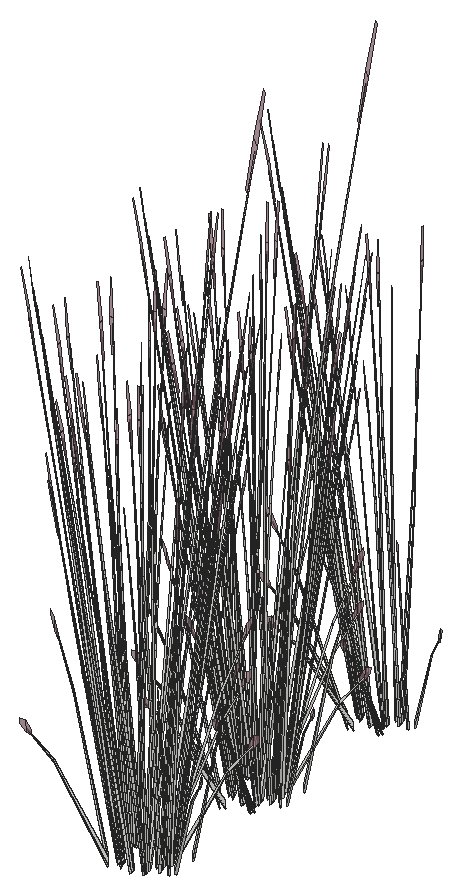
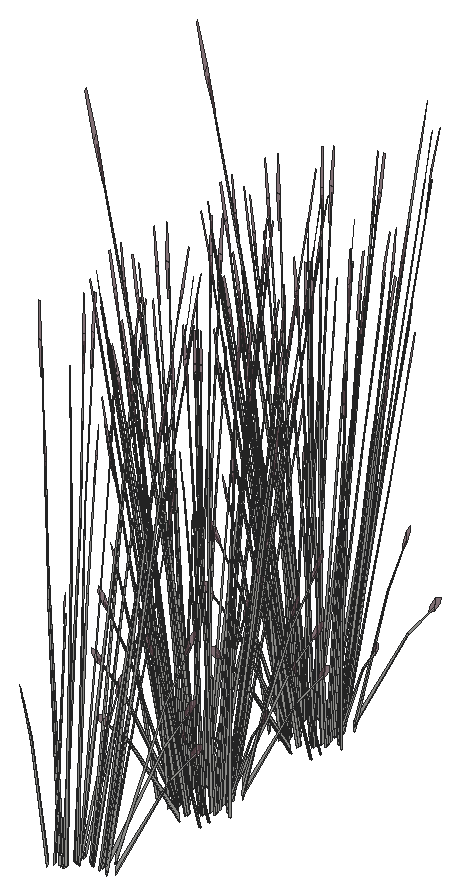
# SketchUp Ruby script. Lengths in inches.
U = 1.inch
M = Sketchup.active_model
def pt(a) = Geom::Point3d.new(a.map { |v| v * U })
def face(e, loops, mat)
  f = e.add_face(loops[0].map { |a| pt(a) })
  loops[1..].each { |l| e.add_face(l.map { |a| pt(a) }).erase! }
  f.material = f.back_material = mat if mat
  f
end
# faces: each face lists its corners as indices into pts; further lists are holes
def faces(e, pts, list, mat = nil) = list.each { |f| face(e, (f[0].is_a?(Array) ? f : [f]).map { |l| l.map { |i| pts[i] } }, mat) }
# xy, xz, yz: faces in a plane at the given z, y or x. An outline is a flat list of corners, or four numbers for a rectangle; further outlines are holes
def ring(l) = l.size == 4 ? [[l[0], l[1]], [l[2], l[1]], [l[2], l[3]], [l[0], l[3]]] : l.each_slice(2).to_a
def flat(e, list, mat, &to3) = list.each { |f| face(e, (f[0].is_a?(Array) ? f : [f]).map { |l| ring(l).map { |u, v| to3.(u, v) } }, mat) }
def xy(e, z, list, mat = nil) = flat(e, list, mat) { |x, y| [x, y, z] }
def xz(e, y, list, mat = nil) = flat(e, list, mat) { |x, z| [x, y, z] }
def yz(e, x, list, mat = nil) = flat(e, list, mat) { |y, z| [x, y, z] }
def lines(e, pts, list) = list.each { |a, b| e.add_line(pt(pts[a]), pt(pts[b])) }
# prism: a flat outline (further loops are holes) pulled along v
def prism(e, loops, v, mat = nil)
  f = face(e, loops, mat); d = Geom::Vector3d.new(v.map { |x| x * U })
  f.pushpull(f.normal.samedirection?(d) ? d.length : -d.length)
end
def box(e, o, s, mat = nil) = prism(e, [[o, [o[0] + s[0], o[1], o[2]], [o[0] + s[0], o[1] + s[1], o[2]], [o[0], o[1] + s[1], o[2]]]], [0, 0, s[2]], mat)
def at(x, y, z, deg = 0) = Geom::Transformation.translation(pt([x, y, z])) * Geom::Transformation.rotation(ORIGIN, Z_AXIS, deg.degrees)
def axes(o, x, y, z) = Geom::Transformation.new([*x, 0, *y, 0, *z, 0, *pt(o).to_a, 1])
def part(name) = M.definitions.add(name)
# library, detail: a bought-in or finely detailed component or shape, given as its bounding box
def library(name, o, s) = part(name).tap { |d| box(d.entities, o, s) }
def detail(e, o, s) = box(e.add_group.entities, o, s)
def put(e, d, t, mat = nil) = e.add_instance(d, t).tap { |i| i.material = mat if mat }
def group(e, t, mat = nil) = e.add_group.tap { |g| g.transformation = t; g.material = mat if mat }.entities
root = M.entities
M.materials.add("LightPink_Translucent").color = [144, 107, 117]
M.materials["LightPink_Translucent"].alpha = 0.75
c1 = part("blade")
p = [[2.15,0.21,22],[0,0.17,0],[0.09,0.45,0],[2.18,0.31,22],[2.29,0.31,22],[0.38,0.45,0],
  [2.48,0.24,33],[2.49,0.24,33],[2.48,0.22,33]]
faces(c1.entities,p,[[0,1,2,3],[4,5,2,3],[6,3,4,7],[8,0,3,6]])
c2 = part("seeds")
p = [[0.3,-0.1,1.38],[-0.01,-0.03,1.59],[-0.01,-0.03,0.03],[0.14,-0.07,-0.07],[0.29,-0.03,3],[0.15,0.01,3.11]]
faces(c2.entities,p,[[0,1,2,3],[1,0,4,5]],"LightPink_Translucent")
c3 = part("blade with seeds")
put(c3.entities,c1,at(0,0,0))
put(c3.entities,c2,axes([2.4,0.25,30.99],[1.5799,-0.05474,1.17369],[-0.12525,1.92788,0.29478],[-0.07173,-0.02425,1.56792]))
put(root,c3,axes([401.45,752.64,5.09],[0.39316,-0.11987,0.53763],[0.06823,0.47021,0.4433],[-0.09247,-0.13858,1.11249]))
put(root,c3,axes([402.34,752.73,4.73],[0.34777,0.12192,0.48003],[-0.11892,0.40083,0.3958],[-0.0209,-0.15763,0.9933]))
put(root,c3,axes([402.4375,752.87,5.03],[-0.34538,0.21713,-0.1216],[-0.16972,-0.38536,-0.67495],[-0.04557,-0.16239,1.02557]))
put(root,c3,axes([403.15,753.36,5.03],[-0.3879,-0.02311,-0.1216],[0.0106,-0.43749,-0.67495],[0.02694,-0.1685,1.02557]))
put(root,c3,axes([402.43,752.69,4.73],[0.26007,-0.1585,0.0643],[0.12729,0.28902,0.50621],[-0.02512,-0.1274,0.77189]))
put(root,c3,axes([401.54,752.74,4.73],[0.16041,-0.29625,0.0643],[0.22843,0.17248,0.50621],[-0.07385,-0.09498,0.77189]))
put(root,c3,axes([402.33,753.02,5.05],[-0.1064,0.35863,0.35414],[-0.31043,-0.1046,-0.4572],[-0.02846,-0.14439,0.87481]))
put(root,c3,axes([403.125,753.17,4.73],[0.25132,0.3182,0.48003],[-0.2669,0.27442,0.3958],[0.04636,-0.14929,0.9933]))
put(root,c3,axes([401.61,752.71,5.43],[-0.23555,0.44708,-0.13619],[-0.34112,-0.25757,-0.75594],[-0.11858,-0.12631,1.14864]))
put(root,c3,axes([403.22,753.2,4.73],[0.29004,0.02173,0.0643],[-0.00795,0.32812,0.50621],[0.03035,-0.12569,0.77189]))
put(root,c3,axes([403,753.42,5.05],[-0.23881,0.24554,0.35414],[-0.22606,-0.28036,-0.4572],[0.0344,-0.14245,0.87481]))
put(root,c3,axes([400.71,752.58,4.72],[-0.07594,-0.00329,1.74944],[-0.24177,0.32918,-0.27667],[-0.129,-0.06726,0.14031]))
put(root,c3,axes([403.58,754.22,5.03],[-0.32648,-0.25715,-0.1216],[0.18809,-0.3724,-0.67495],[0.09224,-0.12945,1.02557]))
put(root,c3,axes([401.59,753.08,5.05],[0.05451,0.37564,0.35414],[-0.31161,0.09919,-0.4572],[-0.0837,-0.10765,0.87481]))
put(root,c3,axes([400.65,753.32,5.09],[0.29147,-0.34417,0.53763],[0.25138,0.3655,0.4433],[-0.13675,-0.06349,1.11249]))
put(root,c3,axes([404.38,754.11,4.71],[-0.0461,-0.00354,1.77383],[-0.19143,-0.37951,-0.16761],[0.07688,-0.12478,0.31391]))
put(root,c3,axes([400.78,753.32,4.73],[0.01777,-0.35463,0.0643],[0.26836,0.00972,0.50621],[-0.1028,-0.03711,0.77189]))
put(root,c3,axes([403.42,754.18,5.05],[-0.30722,0.06665,0.35414],[-0.08112,-0.381,-0.4572],[0.08804,-0.10234,0.87481]))
put(root,c3,axes([403.7,754.12,4.73],[0.2423,0.19613,0.0643],[-0.14107,0.2793,0.50621],[0.07768,-0.0903,0.77189]))
put(root,c3,axes([403.63,754.04,4.73],[0.08753,0.42921,0.48003],[-0.34336,0.07449,0.3958],[0.1012,-0.10094,0.9933]))
put(root,c3,axes([404.55,754.56,4.72],[0.04898,-0.07104,1.74944],[-0.06269,-0.43574,-0.27667],[0.12289,-0.08262,0.14031]))
put(root,c3,axes([400.42,752.86,4.71],[0.02617,0.04654,1.77383],[-0.12614,0.41836,-0.16761],[-0.12775,0.00303,0.31391]))
put(root,c3,axes([400.97,753.59,5.05],[0.20082,0.29199,0.35414],[-0.2293,0.2764,-0.4572],[-0.1165,-0.04206,0.87481]))
put(root,c3,axes([400.91,753.4,5.03],[-0.0189,0.47427,-0.1216],[-0.35781,-0.01296,-0.67495],[-0.13781,-0.03295,1.02557]))
put(root,c3,axes([403.59,755.22,5.03],[-0.17758,-0.42229,-0.1216],[0.31518,-0.20752,-0.67495],[0.13282,-0.05572,1.02557]))
put(root,c3,axes([403.47,755.09,5.05],[-0.29332,-0.1301,0.35414],[0.08555,-0.37955,-0.4572],[0.11809,-0.0348,0.87481]))
put(root,c3,axes([400.4,754.4,4.73],[0.09971,-0.42522,0.48003],[0.32782,0.1454,0.3958],[-0.12892,0.02555,0.9933]))
put(root,c3,axes([400.37,754.29,4.73],[-0.12963,-0.31798,0.0643],[0.23638,-0.15564,0.50621],[-0.1042,0.03071,0.77189]))
put(root,c3,axes([403.73,755.21,4.73],[0.12963,0.31798,0.0643],[-0.23638,0.15564,0.50621],[0.1042,-0.03071,0.77189]))
put(root,c3,axes([403.71,755.1,4.73],[-0.09971,0.42522,0.48003],[-0.32782,-0.1454,0.3958],[0.12892,-0.02555,0.9933]))
put(root,c3,axes([400.64,754.41,5.05],[0.29332,0.1301,0.35414],[-0.08555,0.37955,-0.4572],[-0.11809,0.0348,0.87481]))
put(root,c3,axes([404.3,756.48,4.71],[-0.03191,-0.04083,1.77383],[0.06981,-0.43764,-0.16761],[0.12571,-0.02796,0.31391]))
put(root,c3,axes([400.14,754.7,4.72],[-0.05763,0.06055,1.74944],[0.0049,0.44239,-0.27667],[-0.13211,0.05753,0.14031]))
put(root,c3,axes([400.51,754.28,5.03],[0.17758,0.42229,-0.1216],[-0.31518,0.20752,-0.67495],[-0.13282,0.05572,1.02557]))
put(root,c3,axes([403.19,756.1,5.03],[0.0189,-0.47427,-0.1216],[0.35781,0.01296,-0.67495],[0.13781,0.03295,1.02557]))
put(root,c3,axes([403.14,755.91,5.05],[-0.20082,-0.29199,0.35414],[0.2293,-0.2764,-0.4572],[0.1165,0.04206,0.87481]))
put(root,c3,axes([403.5,755.8125,4.72],[0.07571,-0.00789,1.74944],[0.20767,-0.36231,-0.27667],[0.13467,0.04783,0.14031]))
put(root,c3,axes([400.47,755.46,4.73],[-0.08753,-0.42921,0.48003],[0.34336,-0.07449,0.3958],[-0.1012,0.10094,0.9933]))
put(root,c3,axes([400.41,755.38,4.73],[-0.2423,-0.19613,0.0643],[0.14107,-0.2793,0.50621],[-0.07768,0.0903,0.77189]))
put(root,c3,axes([400.6875,755.32,5.05],[0.30722,-0.06665,0.35414],[0.08112,0.381,-0.4572],[-0.08804,0.10234,0.87481]))
put(root,c3,axes([399.5,755.15,4.71],[0.04504,0.01251,1.77383],[0.13934,0.41205,-0.16761],[-0.0922,0.10815,0.31391]))
put(root,c3,axes([403.32,756.18,4.73],[-0.01777,0.35463,0.0643],[-0.26836,-0.00972,0.50621],[0.1028,0.03711,0.77189]))
put(root,c3,axes([403.34,756.06,4.73],[-0.26024,0.30729,0.48003],[-0.22444,-0.32634,0.3958],[0.1221,0.05668,0.9933]))
put(root,c3,axes([399.99,756.4,5.65],[0.31145,0.12449,-0.06488],[-0.0958,0.38314,-0.29416],[-0.05094,0.05817,0.97024]))
put(root,c3,axes([402.52,756.42,5.05],[-0.05451,-0.37564,0.35414],[0.31161,-0.09919,-0.4572],[0.0837,0.10765,0.87481]))
put(root,c3,axes([402.72,754.26,4.47],[-0.30498,-0.24231,1.38283],[0.32203,-0.37727,0.59665],[0.0984,0.22736,1.33663]))
put(root,c3,axes([400.53,755.28,5.03],[0.32648,0.25715,-0.1216],[-0.18809,0.3724,-0.67495],[-0.09224,0.12945,1.02557]))
put(root,c3,axes([402.49,756.61,5.03],[0.21031,-0.39918,-0.1216],[0.30457,0.22997,-0.67495],[0.10587,0.11278,1.02557]))
put(root,c3,axes([401.1,756.08,5.05],[0.23881,-0.24554,0.35414],[0.22606,0.28036,-0.4572],[-0.0344,0.14245,0.87481]))
put(root,c3,axes([402.21,756.95,4.71],[0.00104,-0.05646,1.77383],[0.30246,-0.2491,-0.16761],[0.10506,0.08891,0.31391]))
put(root,c3,axes([400.88,756.3,4.73],[-0.29004,-0.02173,0.0643],[0.00795,-0.32812,0.50621],[-0.03035,0.12569,0.77189]))
put(root,c3,axes([400.98,756.33,4.73],[-0.25132,-0.3182,0.48003],[0.2669,-0.27442,0.3958],[-0.04636,0.14929,0.9933]))
put(root,c3,axes([401.77,756.48,5.05],[0.1064,-0.35863,0.35414],[0.31043,0.1046,-0.4572],[0.02846,0.14439,0.87481]))
put(root,c3,axes([402.56,756.76,4.73],[-0.16041,0.29625,0.0643],[-0.22843,-0.17248,0.50621],[0.07385,0.09498,0.77189]))
put(root,c3,axes([402.1875,757.76,5.65],[0.2439,-0.26754,-0.06488],[0.22348,0.29302,-0.29416],[0.01573,0.08303,0.97024]))
put(root,c3,axes([402.63,756.68,4.73],[-0.35104,0.10702,0.48003],[-0.06092,-0.41983,0.3958],[0.08256,0.12373,0.9933]))
put(root,c3,axes([401.67,756.8,4.73],[-0.26007,0.1585,0.0643],[-0.12729,-0.28902,0.50621],[0.02512,0.1274,0.77189]))
put(root,c3,axes([400.15,756.35,4.72],[-0.00877,0.09229,1.74944],[0.24897,0.32105,-0.27667],[-0.06518,0.15182,0.14031]))
put(root,c3,axes([400.95,756.14,5.4],[0.3879,0.02311,-0.13498],[-0.0106,0.43749,-0.74919],[-0.02694,0.1685,1.13838]))
put(root,c3,axes([401.67,756.63,5.03],[0.34538,-0.21713,-0.1216],[0.16972,0.38536,-0.67495],[0.04557,0.16239,1.02557]))
put(root,c3,axes([401.77,756.77,5.0625],[-0.34777,-0.12192,0.53283],[0.11892,-0.40083,0.43934],[0.0209,0.15763,1.10256]))
put(root,c3,axes([401.89,762.66,4.72],[-0.05398,-0.06539,1.74944],[-0.36026,0.04145,-0.27667],[-0.0575,-0.15639,0.14031]))
put(root,c3,axes([400.125,757.3,4.71],[0.04004,-0.02816,1.77383],[0.33095,0.18728,-0.16761],[-0.00778,0.15594,0.31391]))
put(root,c3,axes([403.51,763.46,4.72],[-0.00341,-0.09282,1.74944],[-0.28775,-0.26825,-0.27667],[0.04449,-0.16261,0.14031]))
put(root,c3,axes([403.43,763.13,4.71],[-0.03584,0.03562,1.77383],[-0.35118,-0.12018,-0.16761],[-0.01271,-0.15545,0.31391]))
put(root,c3,axes([401.58,757.49,4.72],[0.04474,0.0751,1.74944],[0.36104,0.0295,-0.27667],[0.03631,0.16562,0.14031]))
put(root,c3,axes([401.52,762.45,4.71],[-0.00658,0.0559,1.77383],[-0.32474,0.20287,-0.16761],[-0.09556,-0.1037,0.31391]))
put(root,c3,axes([401.45,763.44,5.09],[0.39316,-0.11987,0.53763],[0.06823,0.47021,0.4433],[-0.09247,-0.13858,1.11249]))
put(root,c3,axes([402.34,763.53,4.73],[0.34777,0.12192,0.48003],[-0.11892,0.40083,0.3958],[-0.0209,-0.15763,0.9933]))
put(root,c3,axes([402.4375,763.67,5.03],[-0.34538,0.21713,-0.1216],[-0.16972,-0.38536,-0.67495],[-0.04557,-0.16239,1.02557]))
put(root,c3,axes([403.15,764.16,5.03],[-0.3879,-0.02311,-0.1216],[0.0106,-0.43749,-0.67495],[0.02694,-0.1685,1.02557]))
put(root,c3,axes([402.43,763.5,4.73],[0.26007,-0.1585,0.0643],[0.12729,0.28902,0.50621],[-0.02512,-0.1274,0.77189]))
put(root,c3,axes([401.54,763.54,4.73],[0.16041,-0.29625,0.0643],[0.22843,0.17248,0.50621],[-0.07385,-0.09498,0.77189]))
put(root,c3,axes([402.33,763.82,5.05],[-0.1064,0.35863,0.35414],[-0.31043,-0.1046,-0.4572],[-0.02846,-0.14439,0.87481]))
put(root,c3,axes([403.125,763.97,4.73],[0.25132,0.3182,0.48003],[-0.2669,0.27442,0.3958],[0.04636,-0.14929,0.9933]))
put(root,c3,axes([401.61,763.51,5.43],[-0.23555,0.44708,-0.13619],[-0.34112,-0.25757,-0.75594],[-0.11858,-0.12631,1.14864]))
put(root,c3,axes([403.22,764,4.73],[0.29004,0.02173,0.0643],[-0.00795,0.32812,0.50621],[0.03035,-0.12569,0.77189]))
put(root,c3,axes([403,764.23,5.05],[-0.23881,0.24554,0.35414],[-0.22606,-0.28036,-0.4572],[0.0344,-0.14245,0.87481]))
put(root,c3,axes([400.71,763.38,4.72],[-0.07594,-0.00329,1.74944],[-0.24177,0.32918,-0.27667],[-0.129,-0.06726,0.14031]))
put(root,c3,axes([403.58,765.02,5.03],[-0.32648,-0.25715,-0.1216],[0.18809,-0.3724,-0.67495],[0.09224,-0.12945,1.02557]))
put(root,c3,axes([401.59,763.88,5.05],[0.05451,0.37564,0.35414],[-0.31161,0.09919,-0.4572],[-0.0837,-0.10765,0.87481]))
put(root,c3,axes([400.65,764.13,5.09],[0.29147,-0.34417,0.53763],[0.25138,0.3655,0.4433],[-0.13675,-0.06349,1.11249]))
put(root,c3,axes([404.38,764.91,4.71],[-0.0461,-0.00354,1.77383],[-0.19143,-0.37951,-0.16761],[0.07688,-0.12478,0.31391]))
put(root,c3,axes([400.78,764.125,4.73],[0.01777,-0.35463,0.0643],[0.26836,0.00972,0.50621],[-0.1028,-0.03711,0.77189]))
put(root,c3,axes([403.42,764.99,5.05],[-0.30722,0.06665,0.35414],[-0.08112,-0.381,-0.4572],[0.08804,-0.10234,0.87481]))
put(root,c3,axes([403.7,764.93,4.73],[0.2423,0.19613,0.0643],[-0.14107,0.2793,0.50621],[0.07768,-0.0903,0.77189]))
put(root,c3,axes([403.63,764.84,4.73],[0.08753,0.42921,0.48003],[-0.34336,0.07449,0.3958],[0.1012,-0.10094,0.9933]))
put(root,c3,axes([404.55,765.36,4.72],[0.04898,-0.07104,1.74944],[-0.06269,-0.43574,-0.27667],[0.12289,-0.08262,0.14031]))
put(root,c3,axes([400.42,763.66,4.71],[0.02617,0.04654,1.77383],[-0.12614,0.41836,-0.16761],[-0.12775,0.00303,0.31391]))
put(root,c3,axes([400.97,764.39,5.05],[0.20082,0.29199,0.35414],[-0.2293,0.2764,-0.4572],[-0.1165,-0.04206,0.87481]))
put(root,c3,axes([400.91,764.2,5.03],[-0.0189,0.47427,-0.1216],[-0.35781,-0.01296,-0.67495],[-0.13781,-0.03295,1.02557]))
put(root,c3,axes([403.59,766.02,5.03],[-0.17758,-0.42229,-0.1216],[0.31518,-0.20752,-0.67495],[0.13282,-0.05572,1.02557]))
put(root,c3,axes([403.47,765.9,5.05],[-0.29332,-0.1301,0.35414],[0.08555,-0.37955,-0.4572],[0.11809,-0.0348,0.87481]))
put(root,c3,axes([400.4,765.2,4.73],[0.09971,-0.42522,0.48003],[0.32782,0.1454,0.3958],[-0.12892,0.02555,0.9933]))
put(root,c3,axes([400.37,765.09,4.73],[-0.12963,-0.31798,0.0643],[0.23638,-0.15564,0.50621],[-0.1042,0.03071,0.77189]))
put(root,c3,axes([403.73,766.01,4.73],[0.12963,0.31798,0.0643],[-0.23638,0.15564,0.50621],[0.1042,-0.03071,0.77189]))
put(root,c3,axes([403.71,765.9,4.73],[-0.09971,0.42522,0.48003],[-0.32782,-0.1454,0.3958],[0.12892,-0.02555,0.9933]))
put(root,c3,axes([400.64,765.21,5.05],[0.29332,0.1301,0.35414],[-0.08555,0.37955,-0.4572],[-0.11809,0.0348,0.87481]))
put(root,c3,axes([404.3,767.28,4.71],[-0.03191,-0.04083,1.77383],[0.06981,-0.43764,-0.16761],[0.12571,-0.02796,0.31391]))
put(root,c3,axes([400.14,765.5,4.72],[-0.05763,0.06055,1.74944],[0.0049,0.44239,-0.27667],[-0.13211,0.05753,0.14031]))
put(root,c3,axes([400.51,765.08,5.03],[0.17758,0.42229,-0.1216],[-0.31518,0.20752,-0.67495],[-0.13282,0.05572,1.02557]))
put(root,c3,axes([403.19,766.9,5.03],[0.0189,-0.47427,-0.1216],[0.35781,0.01296,-0.67495],[0.13781,0.03295,1.02557]))
put(root,c3,axes([403.14,766.72,5.05],[-0.20082,-0.29199,0.35414],[0.2293,-0.2764,-0.4572],[0.1165,0.04206,0.87481]))
put(root,c3,axes([403.5,766.62,4.72],[0.07571,-0.00789,1.74944],[0.20767,-0.36231,-0.27667],[0.13467,0.04783,0.14031]))
put(root,c3,axes([400.47,766.26,4.73],[-0.08753,-0.42921,0.48003],[0.34336,-0.07449,0.3958],[-0.1012,0.10094,0.9933]))
put(root,c3,axes([400.41,766.18,4.73],[-0.2423,-0.19613,0.0643],[0.14107,-0.2793,0.50621],[-0.07768,0.0903,0.77189]))
put(root,c3,axes([400.6875,766.12,5.05],[0.30722,-0.06665,0.35414],[0.08112,0.381,-0.4572],[-0.08804,0.10234,0.87481]))
put(root,c3,axes([399.5,765.95,4.71],[0.04504,0.01251,1.77383],[0.13934,0.41205,-0.16761],[-0.0922,0.10815,0.31391]))
put(root,c3,axes([403.32,766.98,4.73],[-0.01777,0.35463,0.0643],[-0.26836,-0.00972,0.50621],[0.1028,0.03711,0.77189]))
put(root,c3,axes([403.34,766.87,4.73],[-0.26024,0.30729,0.48003],[-0.22444,-0.32634,0.3958],[0.1221,0.05668,0.9933]))
put(root,c3,axes([399.99,767.2,5.65],[0.31145,0.12449,-0.06488],[-0.0958,0.38314,-0.29416],[-0.05094,0.05817,0.97024]))
put(root,c3,axes([402.52,767.22,5.05],[-0.05451,-0.37564,0.35414],[0.31161,-0.09919,-0.4572],[0.0837,0.10765,0.87481]))
put(root,c3,axes([402.72,765.0625,4.47],[-0.30498,-0.24231,1.38283],[0.32203,-0.37727,0.59665],[0.0984,0.22736,1.33663]))
put(root,c3,axes([400.53,766.08,5.03],[0.32648,0.25715,-0.1216],[-0.18809,0.3724,-0.67495],[-0.09224,0.12945,1.02557]))
put(root,c3,axes([402.49,767.42,5.03],[0.21031,-0.39918,-0.1216],[0.30457,0.22997,-0.67495],[0.10587,0.11278,1.02557]))
put(root,c3,axes([401.1,766.88,5.05],[0.23881,-0.24554,0.35414],[0.22606,0.28036,-0.4572],[-0.0344,0.14245,0.87481]))
put(root,c3,axes([402.21,767.75,4.71],[0.00104,-0.05646,1.77383],[0.30246,-0.2491,-0.16761],[0.10506,0.08891,0.31391]))
put(root,c3,axes([400.88,767.1,4.73],[-0.29004,-0.02173,0.0643],[0.00795,-0.32812,0.50621],[-0.03035,0.12569,0.77189]))
put(root,c3,axes([400.98,767.13,4.73],[-0.25132,-0.3182,0.48003],[0.2669,-0.27442,0.3958],[-0.04636,0.14929,0.9933]))
put(root,c3,axes([401.77,767.28,5.05],[0.1064,-0.35863,0.35414],[0.31043,0.1046,-0.4572],[0.02846,0.14439,0.87481]))
put(root,c3,axes([402.56,767.5625,4.73],[-0.16041,0.29625,0.0643],[-0.22843,-0.17248,0.50621],[0.07385,0.09498,0.77189]))
put(root,c3,axes([402.1875,768.5625,5.65],[0.2439,-0.26754,-0.06488],[0.22348,0.29302,-0.29416],[0.01573,0.08303,0.97024]))
put(root,c3,axes([402.63,767.48,4.73],[-0.35104,0.10702,0.48003],[-0.06092,-0.41983,0.3958],[0.08256,0.12373,0.9933]))
put(root,c3,axes([401.67,767.61,4.73],[-0.26007,0.1585,0.0643],[-0.12729,-0.28902,0.50621],[0.02512,0.1274,0.77189]))
put(root,c3,axes([400.15,767.15,4.72],[-0.00877,0.09229,1.74944],[0.24897,0.32105,-0.27667],[-0.06518,0.15182,0.14031]))
put(root,c3,axes([400.95,766.95,5.4],[0.3879,0.02311,-0.13498],[-0.0106,0.43749,-0.74919],[-0.02694,0.1685,1.13838]))
put(root,c3,axes([401.67,767.43,5.03],[0.34538,-0.21713,-0.1216],[0.16972,0.38536,-0.67495],[0.04557,0.16239,1.02557]))
put(root,c3,axes([401.77,767.58,5.0625],[-0.34777,-0.12192,0.53283],[0.11892,-0.40083,0.43934],[0.0209,0.15763,1.10256]))
put(root,c3,axes([400.125,768.1,4.71],[0.04004,-0.02816,1.77383],[0.33095,0.18728,-0.16761],[-0.00778,0.15594,0.31391]))
put(root,c3,axes([401.58,768.3,4.72],[0.04474,0.0751,1.74944],[0.36104,0.0295,-0.27667],[0.03631,0.16562,0.14031]))
put(root,c3,axes([401.89,775.04,4.72],[-0.05398,-0.06539,1.74944],[-0.36026,0.04145,-0.27667],[-0.0575,-0.15639,0.14031]))
put(root,c3,axes([403.51,775.84,4.72],[-0.00341,-0.09282,1.74944],[-0.28775,-0.26825,-0.27667],[0.04449,-0.16261,0.14031]))
put(root,c3,axes([403.43,775.51,4.71],[-0.03584,0.03562,1.77383],[-0.35118,-0.12018,-0.16761],[-0.01271,-0.15545,0.31391]))
put(root,c3,axes([401.52,774.83,4.71],[-0.00658,0.0559,1.77383],[-0.32474,0.20287,-0.16761],[-0.09556,-0.1037,0.31391]))
put(root,c3,axes([401.45,775.82,5.09],[0.39316,-0.11987,0.53763],[0.06823,0.47021,0.4433],[-0.09247,-0.13858,1.11249]))
put(root,c3,axes([402.34,775.91,4.73],[0.34777,0.12192,0.48003],[-0.11892,0.40083,0.3958],[-0.0209,-0.15763,0.9933]))
put(root,c3,axes([402.4375,776.05,5.03],[-0.34538,0.21713,-0.1216],[-0.16972,-0.38536,-0.67495],[-0.04557,-0.16239,1.02557]))
put(root,c3,axes([403.15,776.54,5.03],[-0.3879,-0.02311,-0.1216],[0.0106,-0.43749,-0.67495],[0.02694,-0.1685,1.02557]))
put(root,c3,axes([402.43,775.875,4.73],[0.26007,-0.1585,0.0643],[0.12729,0.28902,0.50621],[-0.02512,-0.1274,0.77189]))
put(root,c3,axes([401.54,775.92,4.73],[0.16041,-0.29625,0.0643],[0.22843,0.17248,0.50621],[-0.07385,-0.09498,0.77189]))
put(root,c3,axes([402.33,776.2,5.05],[-0.1064,0.35863,0.35414],[-0.31043,-0.1046,-0.4572],[-0.02846,-0.14439,0.87481]))
put(root,c3,axes([403.125,776.35,4.73],[0.25132,0.3182,0.48003],[-0.2669,0.27442,0.3958],[0.04636,-0.14929,0.9933]))
put(root,c3,axes([401.61,775.89,5.43],[-0.23555,0.44708,-0.13619],[-0.34112,-0.25757,-0.75594],[-0.11858,-0.12631,1.14864]))
put(root,c3,axes([403.22,776.38,4.73],[0.29004,0.02173,0.0643],[-0.00795,0.32812,0.50621],[0.03035,-0.12569,0.77189]))
put(root,c3,axes([403,776.6,5.05],[-0.23881,0.24554,0.35414],[-0.22606,-0.28036,-0.4572],[0.0344,-0.14245,0.87481]))
put(root,c3,axes([400.71,775.76,4.72],[-0.07594,-0.00329,1.74944],[-0.24177,0.32918,-0.27667],[-0.129,-0.06726,0.14031]))
put(root,c3,axes([403.58,777.4,5.03],[-0.32648,-0.25715,-0.1216],[0.18809,-0.3724,-0.67495],[0.09224,-0.12945,1.02557]))
put(root,c3,axes([401.59,776.26,5.05],[0.05451,0.37564,0.35414],[-0.31161,0.09919,-0.4572],[-0.0837,-0.10765,0.87481]))
put(root,c3,axes([400.65,776.5,5.09],[0.29147,-0.34417,0.53763],[0.25138,0.3655,0.4433],[-0.13675,-0.06349,1.11249]))
put(root,c3,axes([404.38,777.29,4.71],[-0.0461,-0.00354,1.77383],[-0.19143,-0.37951,-0.16761],[0.07688,-0.12478,0.31391]))
put(root,c3,axes([400.78,776.5,4.73],[0.01777,-0.35463,0.0643],[0.26836,0.00972,0.50621],[-0.1028,-0.03711,0.77189]))
put(root,c3,axes([403.42,777.36,5.05],[-0.30722,0.06665,0.35414],[-0.08112,-0.381,-0.4572],[0.08804,-0.10234,0.87481]))
put(root,c3,axes([403.7,777.3,4.73],[0.2423,0.19613,0.0643],[-0.14107,0.2793,0.50621],[0.07768,-0.0903,0.77189]))
put(root,c3,axes([403.63,777.22,4.73],[0.08753,0.42921,0.48003],[-0.34336,0.07449,0.3958],[0.1012,-0.10094,0.9933]))
put(root,c3,axes([404.55,777.74,4.72],[0.04898,-0.07104,1.74944],[-0.06269,-0.43574,-0.27667],[0.12289,-0.08262,0.14031]))
